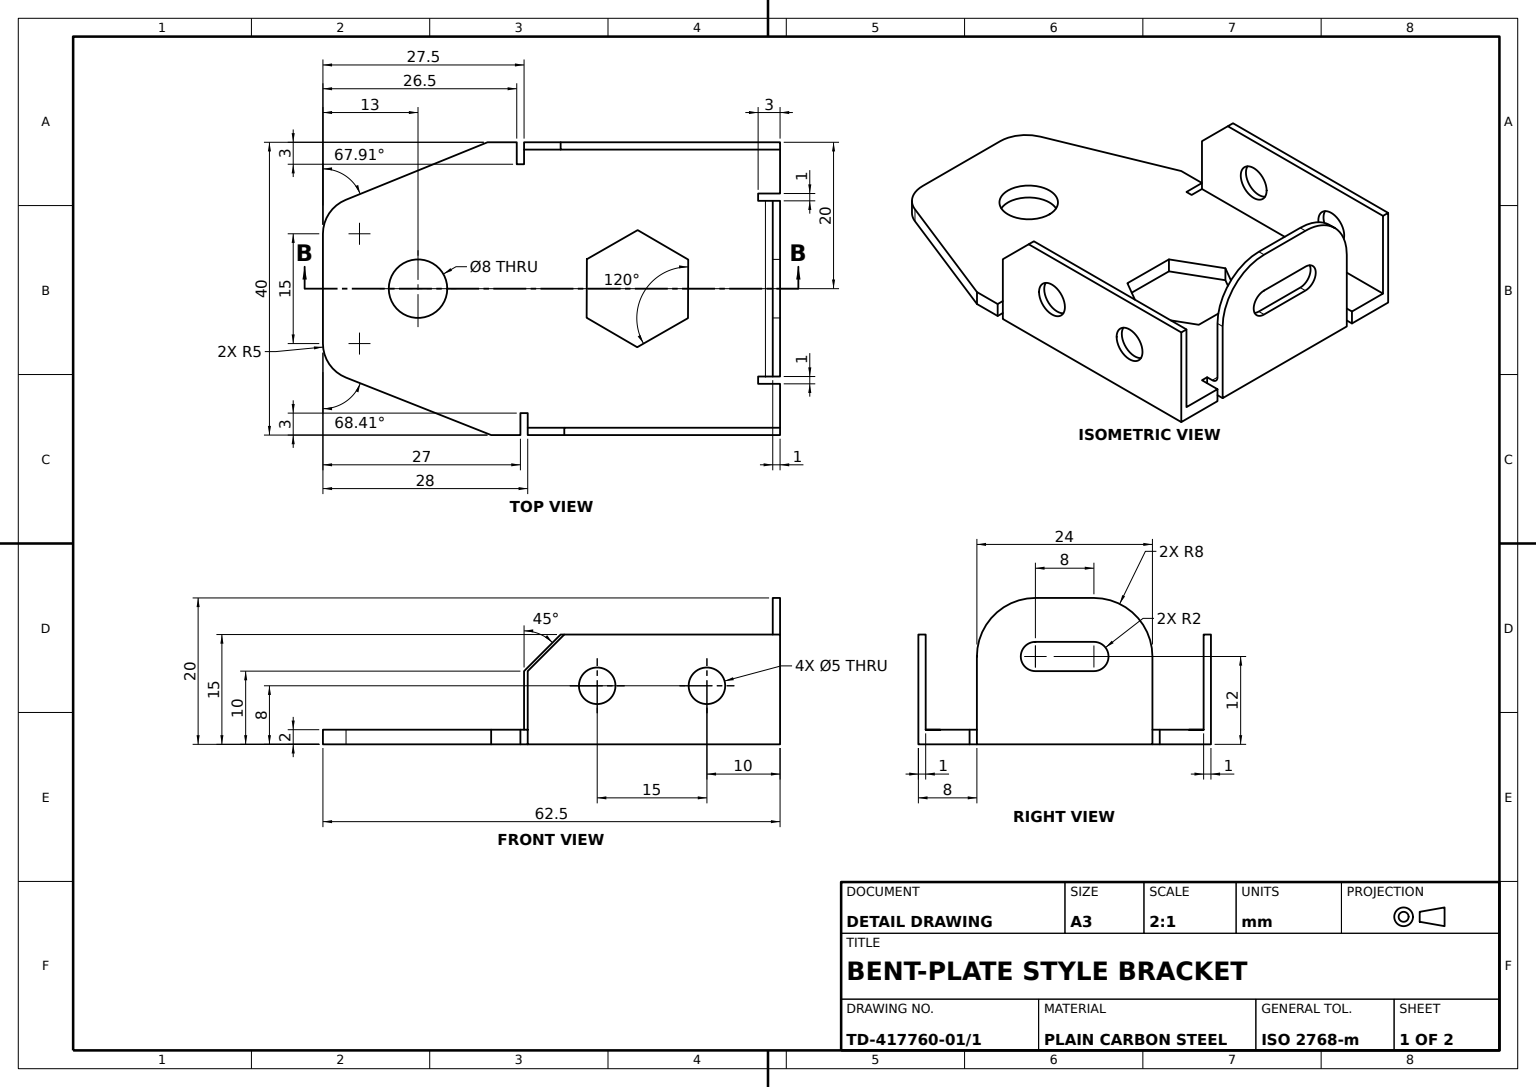
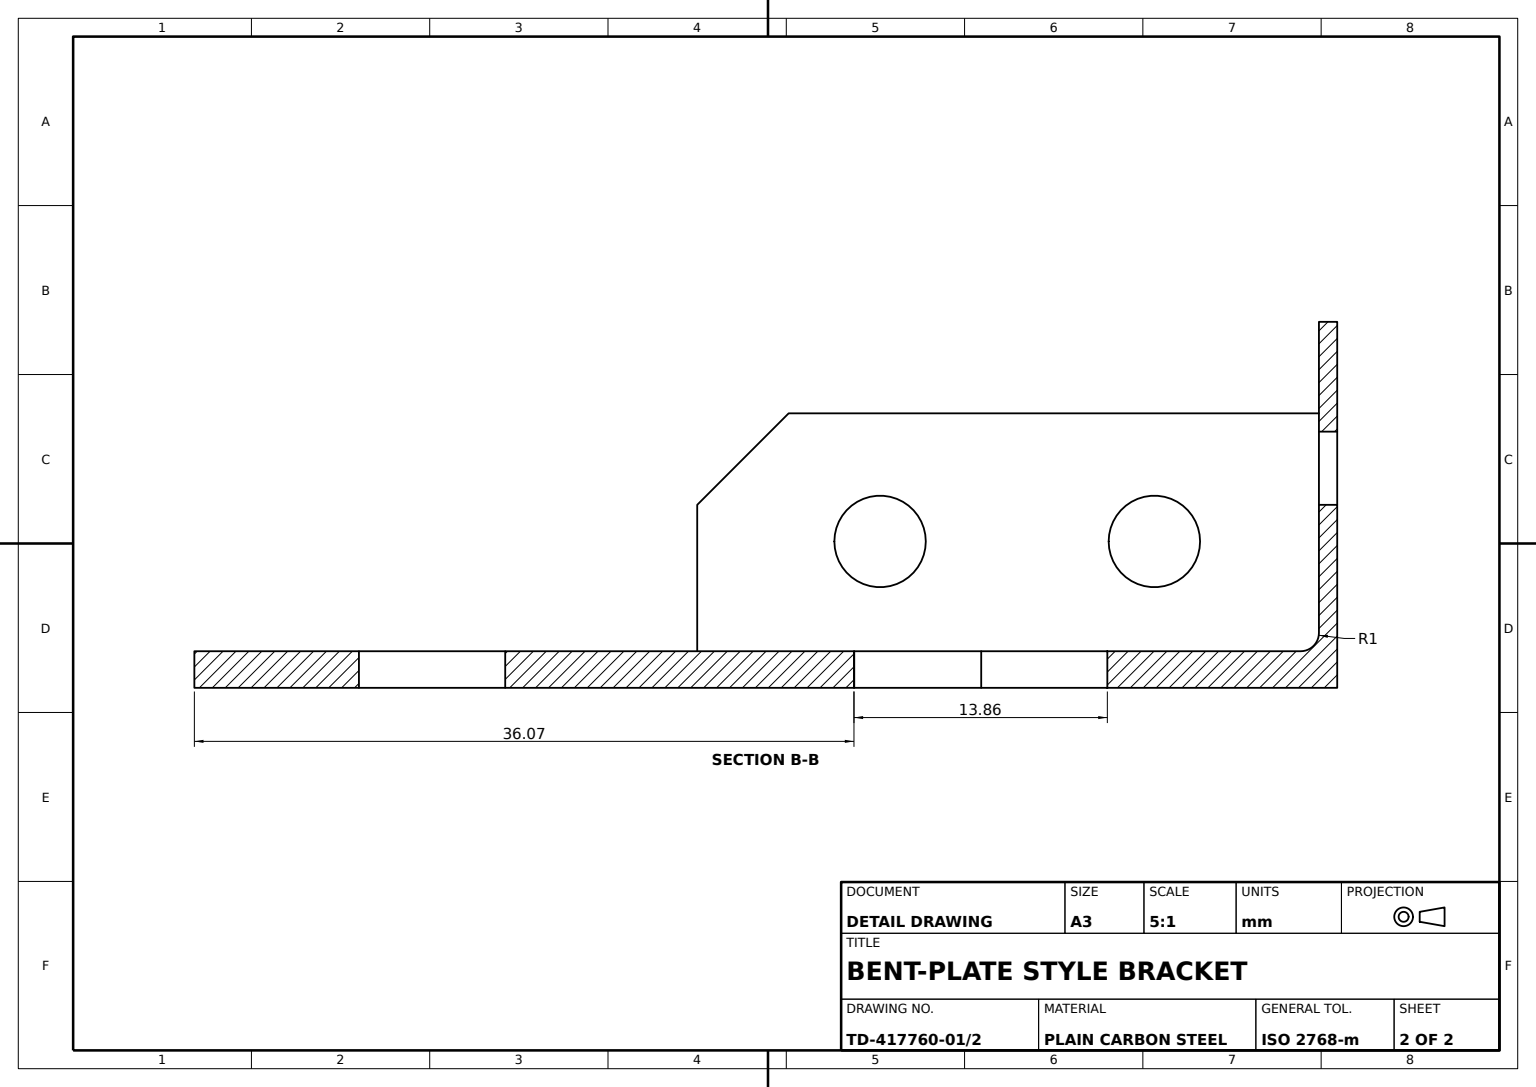
solid
v1 (4,20,1)
v2 (4,20,0)
e1 v1 v2 LINE
v3 (12,12,1)
e2 v3 v1 CIRCLE(AX(P(4,12,1),D(0,0,1),D(1,0,0)),8)
v4 (12,12,0)
e3 v4 v3 LINE
e4 v2 v4 CIRCLE(AX(P(4,12,0),D(0,0,-1),D(-1,0,0)),8)
face CYL(AX(P(4,12,1),D(0,0,-1),D(-1,0,0)),8) [-e1 -e2 -e3 -e4]
v5 (-3.99888,14,0)
v6 (3.99888,14,0)
e5 v5 v6 LINE
v7 (3.99888,14,1)
e6 v6 v7 LINE
v8 (-3.99888,14,1)
e7 v7 v8 LINE
e8 v5 v8 LINE
face PLANE(AX(P(-3.99888,14,-1),D(0,1,0),D(0,0,1))) rev [e5 e6 e7 -e8]
v9 (-19,2,35)
v10 (-17,2,35)
e9 v9 v10 LINE
v11 (-19,10,35)
e10 v9 v11 LINE
v12 (-20,10,35)
e11 v11 v12 LINE
v13 (-20,0,35)
e12 v12 v13 LINE
v14 (-17,0,35)
e13 v13 v14 LINE
e14 v10 v14 LINE
face PLANE(AX(P(0,2,35),D(0,0,-1),D(-1,0,0))) rev [-e9 e10 e11 e12 e13 -e14]
v15 (0,2,53.5)
v16 (0,2,45.5)
e15 v15 v16 CIRCLE(AX(P(0,2,49.5),D(0,1,0),D(0,0,1)),4)
v17 (0,0,45.5)
e16 v16 v17 LINE
v18 (0,0,53.5)
e17 v18 v17 CIRCLE(AX(P(0,0,49.5),D(0,1,0),D(0,0,1)),4)
e18 v15 v18 LINE
face CYL(AX(P(0,2,49.5),D(0,-1,0),D(0,0,-1)),4) rev [e15 e16 -e17 -e18]
v19 (3.973244,2,26.443651)
v20 (8,2,19.530895)
e19 v19 v20 LINE
v21 (8,0,19.530895)
e20 v20 v21 LINE
v22 (3.973244,0,26.443651)
e21 v22 v21 LINE
e22 v19 v22 LINE
face PLANE(AX(P(14.467771,2,8.427635),D(-0.864088023,0,-0.503340728),D(-0.503340728,0,0.864088023))) [e19 e20 -e21 -e22]
v23 (-20,8,27.5)
v24 (-20,8,22.5)
e23 v23 v24 CIRCLE(AX(P(-20,8,25),D(-1,0,0),D(0,0,1)),2.5)
e24 v24 v23 CIRCLE(AX(P(-20,8,25),D(-1,0,0),D(0,0,1)),2.5)
v25 (-20,8,12.5)
v26 (-20,8,7.5)
e25 v25 v26 CIRCLE(AX(P(-20,8,10),D(-1,0,0),D(0,0,1)),2.5)
e26 v26 v25 CIRCLE(AX(P(-20,8,10),D(-1,0,0),D(0,0,1)),2.5)
v27 (-20,15,0)
v28 (-20,0,0)
e27 v27 v28 LINE
e28 v28 v13 LINE
v29 (-20,15,30)
e29 v12 v29 LINE
e30 v29 v27 LINE
face PLANE(AX(P(-20,2,0),D(1,0,0),D(0,0,-1))) rev [-e23 -e24] [-e25 -e26] [e27 e28 -e12 e29 e30]
v30 (-8,2,19.469105)
v31 (-8,0,19.469105)
e31 v30 v31 LINE
v32 (-4.026756,2,26.412756)
e32 v30 v32 LINE
v33 (-4.026756,0,26.412756)
e33 v32 v33 LINE
e34 v31 v33 LINE
face PLANE(AX(P(-14.419221,2,8.250859),D(0.867949869,0,-0.496651815),D(-0.496651815,0,-0.867949869))) [-e31 e32 e33 -e34]
e35 v16 v15 CIRCLE(AX(P(0,2,49.5),D(0,1,0),D(0,0,1)),4)
e36 v17 v18 CIRCLE(AX(P(0,0,49.5),D(0,1,0),D(0,0,1)),4)
face CYL(AX(P(0,2,49.5),D(0,-1,0),D(0,0,-1)),4) rev [e35 e18 -e36 -e16]
v34 (20,15,0)
v35 (20,0,0)
e37 v34 v35 LINE
v36 (13,0,0)
e38 v36 v35 LINE
v37 (13,2,0)
e39 v37 v36 LINE
v38 (19,2,0)
e40 v37 v38 LINE
v39 (19,15,0)
e41 v38 v39 LINE
e42 v39 v34 LINE
face PLANE(AX(P(0,2,0),D(0,0,-1),D(-1,0,0))) [e37 -e38 -e39 e40 e41 e42]
v40 (4.026756,0,12.587244)
e43 v21 v40 LINE
v41 (4.026756,2,12.587244)
e44 v20 v41 LINE
e45 v41 v40 LINE
face PLANE(AX(P(-2.392465,2,1.368999),D(-0.867949869,0,0.496651815),D(0.496651815,0,0.867949869))) [-e43 -e20 e44 e45]
v42 (20,8,22.5)
v43 (20,8,27.5)
e46 v42 v43 CIRCLE(AX(P(20,8,25),D(1,0,0),D(0,0,-1)),2.5)
v44 (19,8,27.5)
e47 v43 v44 LINE
v45 (19,8,22.5)
e48 v45 v44 CIRCLE(AX(P(19,8,25),D(1,0,0),D(0,0,-1)),2.5)
e49 v42 v45 LINE
face CYL(AX(P(30,8,25),D(-1,0,0),D(0,0,1)),2.5) rev [e46 e47 -e48 -e49]
v46 (12,2,2)
v47 (12,2,3)
e50 v46 v47 LINE
v48 (-12,2,2)
e51 v46 v48 LINE
v49 (-12,2,3)
e52 v48 v49 LINE
v50 (-13,2,3)
e53 v49 v50 LINE
v51 (-13,2,0)
e54 v50 v51 LINE
v52 (-19,2,0)
e55 v52 v51 LINE
e56 v52 v9 LINE
v53 (-17,2,36)
e57 v10 v53 LINE
v54 (-20,2,36)
e58 v53 v54 LINE
v55 (-20,2,40)
e59 v54 v55 LINE
v56 (-12.132851,2,59.380608)
e60 v56 v55 LINE
v57 (-7.5,2,62.5)
e61 v56 v57 CIRCLE(AX(P(-7.5,2,57.5),D(0,1,0),D(0,0,1)),5)
v58 (7.5,2,62.5)
e62 v57 v58 LINE
v59 (12.14923,2,59.339743)
e63 v58 v59 CIRCLE(AX(P(7.5,2,57.5),D(0,1,0),D(0,0,1)),5)
v60 (20,2,39.5)
e64 v59 v60 LINE
v61 (20,2,35.5)
e65 v61 v60 LINE
v62 (17,2,35.5)
e66 v62 v61 LINE
v63 (17,2,34.5)
e67 v63 v62 LINE
v64 (19,2,34.5)
e68 v64 v63 LINE
e69 v64 v38 LINE
v65 (13,2,3)
e70 v65 v37 LINE
e71 v47 v65 LINE
v66 (-3.973244,2,12.556349)
e72 v66 v30 LINE
e73 v41 v66 LINE
e74 v32 v19 LINE
face PLANE(AX(P(0,2,0),D(0,1,0),D(0,0,1))) [-e50 e51 e52 e53 e54 -e55 e56 e9 e57 e58 e59 -e60 e61 e62 e63 e64 -e65 -e66 -e67 -e68 e69 -e40 -e70 -e71] [-e72 -e73 -e44 -e19 -e74 -e32] [-e35 -e15]
v67 (20,15,29.5)
v68 (20,10,34.5)
e75 v67 v68 LINE
v69 (19,15,29.5)
e76 v69 v67 LINE
v70 (19,10,34.5)
e77 v69 v70 LINE
e78 v70 v68 LINE
face PLANE(AX(P(19,22.25,22.25),D(0,0.707106781,0.707106781),D(0,-0.707106781,0.707106781))) [-e75 -e76 e77 e78]
v71 (-19,8,22.5)
e79 v71 v24 LINE
v72 (-19,8,27.5)
e80 v72 v71 CIRCLE(AX(P(-19,8,25),D(-1,0,0),D(0,0,1)),2.5)
e81 v72 v23 LINE
face CYL(AX(P(30,8,25),D(-1,0,0),D(0,0,1)),2.5) rev [e23 -e79 -e80 e81]
v73 (-4,20,0)
e82 v73 v2 LINE
v74 (-4,20,1)
e83 v73 v74 LINE
e84 v74 v1 LINE
face PLANE(AX(P(12,20,1),D(0,1,0),D(0,0,1))) [-e82 e83 e84 e1]
v75 (-20,0,40)
e85 v55 v75 LINE
v76 (-20,0,36)
e86 v54 v76 LINE
e87 v76 v75 LINE
face PLANE(AX(P(-20,2,0),D(1,0,0),D(0,0,-1))) rev [-e85 -e59 e86 e87]
v77 (20,8,7.5)
v78 (19,8,7.5)
e88 v77 v78 LINE
v79 (20,8,12.5)
e89 v77 v79 CIRCLE(AX(P(20,8,10),D(1,0,0),D(0,0,-1)),2.5)
v80 (19,8,12.5)
e90 v79 v80 LINE
e91 v78 v80 CIRCLE(AX(P(19,8,10),D(1,0,0),D(0,0,-1)),2.5)
face CYL(AX(P(30,8,10),D(-1,0,0),D(0,0,1)),2.5) rev [-e88 e89 e90 -e91]
v81 (12,3,1)
e92 v81 v46 CIRCLE(AX(P(12,3,2),D(-1,0,0),D(0,0,-1)),1)
v82 (-12,3,1)
e93 v82 v81 LINE
e94 v48 v82 CIRCLE(AX(P(-12,3,2),D(1,0,0),D(0,0,-1)),1)
face CYL(AX(P(0,3,2),D(-1,0,0),D(0,0,1)),1) rev [-e51 -e92 -e93 -e94]
e95 v43 v42 CIRCLE(AX(P(20,8,25),D(1,0,0),D(0,0,-1)),2.5)
e96 v79 v77 CIRCLE(AX(P(20,8,10),D(1,0,0),D(0,0,-1)),2.5)
e97 v34 v67 LINE
v83 (20,0,34.5)
e98 v68 v83 LINE
e99 v35 v83 LINE
face PLANE(AX(P(20,2,0),D(1,0,0),D(0,0,-1))) [-e95 -e46] [-e96 -e89] [-e37 e97 e75 e98 -e99]
e100 v44 v45 CIRCLE(AX(P(19,8,25),D(1,0,0),D(0,0,-1)),2.5)
e101 v64 v70 LINE
e102 v39 v69 LINE
e103 v80 v78 CIRCLE(AX(P(19,8,10),D(1,0,0),D(0,0,-1)),2.5)
face PLANE(AX(P(19,0,0),D(1,0,0),D(0,0,-1))) rev [e100 e48] [e101 -e77 -e102 -e41 -e69] [e91 e103]
v84 (-19,8,7.5)
e104 v84 v26 LINE
v85 (-19,8,12.5)
e105 v85 v84 CIRCLE(AX(P(-19,8,10),D(-1,0,0),D(0,0,1)),2.5)
e106 v85 v25 LINE
face CYL(AX(P(30,8,10),D(-1,0,0),D(0,0,1)),2.5) rev [e25 -e104 -e105 e106]
v86 (13,0,3)
e107 v65 v86 LINE
v87 (12,0,3)
e108 v87 v86 LINE
e109 v47 v87 LINE
face PLANE(AX(P(0,2,3),D(0,0,-1),D(-1,0,0))) [e107 -e108 -e109 e71]
v88 (-13,0,3)
v89 (-13,0,0)
e110 v88 v89 LINE
e111 v51 v89 LINE
e112 v50 v88 LINE
face PLANE(AX(P(-13,2,0),D(-1,0,0),D(0,0,1))) rev [e110 -e111 -e54 e112]
v90 (-17,0,36)
e113 v53 v90 LINE
e114 v90 v76 LINE
face PLANE(AX(P(0,2,36),D(0,0,1),D(1,0,0))) rev [e113 e114 -e86 -e58]
v91 (17,0,35.5)
e115 v62 v91 LINE
v92 (17,0,34.5)
e116 v92 v91 LINE
e117 v63 v92 LINE
face PLANE(AX(P(17,2,0),D(1,0,0),D(0,0,-1))) [e115 -e116 -e117 e67]
v93 (20,0,35.5)
e118 v61 v93 LINE
v94 (20,0,39.5)
e119 v60 v94 LINE
e120 v93 v94 LINE
face PLANE(AX(P(20,2,0),D(1,0,0),D(0,0,-1))) [-e118 e65 e119 -e120]
e121 v84 v85 CIRCLE(AX(P(-19,8,10),D(-1,0,0),D(0,0,1)),2.5)
e122 v71 v72 CIRCLE(AX(P(-19,8,25),D(-1,0,0),D(0,0,1)),2.5)
v95 (-19,15,30)
v96 (-19,15,0)
e123 v95 v96 LINE
e124 v11 v95 LINE
e125 v96 v52 LINE
face PLANE(AX(P(-19,0,0),D(-1,0,0),D(0,0,1))) rev [e121 e105] [e80 e122] [-e123 -e124 -e10 -e56 -e125]
v97 (7.5,0,62.5)
e126 v58 v97 LINE
v98 (-7.5,0,62.5)
e127 v57 v98 LINE
e128 v98 v97 LINE
face PLANE(AX(P(0,2,62.5),D(0,0,-1),D(-1,0,0))) rev [-e126 -e62 e127 e128]
v99 (-12,12,1)
e129 v82 v99 LINE
v100 (-12,12,0)
e130 v99 v100 LINE
v101 (-12,0,0)
e131 v101 v100 LINE
v102 (-12,0,3)
e132 v101 v102 LINE
e133 v49 v102 LINE
face PLANE(AX(P(-12,2,0),D(1,0,0),D(0,0,-1))) rev [-e52 e94 e129 e130 -e131 e132 -e133]
e134 v95 v29 LINE
face PLANE(AX(P(-19,10,35),D(0,0.707106781,0.707106781),D(0,-0.707106781,0.707106781))) [e124 e134 -e29 -e11]
e135 v86 v36 LINE
face PLANE(AX(P(13,2,0),D(-1,0,0),D(0,0,1))) [e70 e39 -e135 -e107]
face CYL(AX(P(30,8,10),D(-1,0,0),D(0,0,1)),2.5) rev [-e106 -e121 e104 e26]
v103 (-3.973244,0,12.556349)
e136 v66 v103 LINE
e137 v40 v103 LINE
face PLANE(AX(P(-0.04855,2,12.571506),D(-0.003861845,0,0.999992543),D(0.999992543,0,0.003861845))) [e73 e136 -e137 -e45]
e138 v102 v88 LINE
face PLANE(AX(P(0,2,3),D(0,0,1),D(1,0,0))) rev [e133 e138 -e112 -e53]
e139 v74 v99 CIRCLE(AX(P(-4,12,1),D(0,0,1),D(1,0,0)),8)
e140 v100 v73 CIRCLE(AX(P(-4,12,0),D(0,0,-1),D(-1,0,0)),8)
face CYL(AX(P(-4,12,0),D(0,0,1),D(1,0,0)),8) [-e139 -e83 -e140 -e130]
e141 v14 v90 LINE
face PLANE(AX(P(-17,2,0),D(1,0,0),D(0,0,-1))) rev [e141 -e113 -e57 e14]
v104 (-3.99888,10,0)
v105 (-3.99888,10,1)
e142 v104 v105 LINE
v106 (3.99888,10,1)
e143 v105 v106 LINE
v107 (3.99888,10,0)
e144 v107 v106 LINE
e145 v107 v104 LINE
face PLANE(AX(P(-3.99888,10,-1),D(0,-1,0),D(0,0,-1))) rev [e142 e143 -e144 e145]
v108 (5.99888,12,1)
e146 v108 v7 CIRCLE(AX(P(3.99888,12,1),D(0,0,1),D(1,0,0)),2)
e147 v106 v108 CIRCLE(AX(P(3.99888,12,1),D(0,0,1),D(1,0,0)),2)
e148 v8 v105 CIRCLE(AX(P(-3.99888,12,1),D(0,0,1),D(1,0,0)),2)
e149 v3 v81 LINE
face PLANE(AX(P(0,0,1),D(0,0,1),D(1,0,0))) [-e7 -e146 -e147 -e143 -e148] [e139 -e129 e93 -e149 e2 -e84]
face CYL(AX(P(30,8,25),D(-1,0,0),D(0,0,1)),2.5) rev [e79 e24 -e81 -e122]
e150 v91 v93 LINE
face PLANE(AX(P(0,2,35.5),D(0,0,-1),D(-1,0,0))) [e66 e118 -e150 -e115]
e151 v96 v27 LINE
face PLANE(AX(P(-19,15,30),D(0,1,0),D(0,0,1))) [-e30 -e134 e123 e151]
face CYL(AX(P(30,8,10),D(-1,0,0),D(0,0,1)),2.5) rev [-e90 e96 e88 -e103]
v109 (5.99888,12,0)
e152 v109 v107 CIRCLE(AX(P(3.99888,12,0),D(0,0,-1),D(-1,0,0)),2)
e153 v109 v108 LINE
face CYL(AX(P(3.99888,12,-1),D(0,0,1),D(1,0,0)),2) rev [e152 e144 e147 -e153]
e154 v103 v31 LINE
face PLANE(AX(P(2.494526,2,1.453089),D(0.864088023,0,0.503340728),D(0.503340728,0,-0.864088023))) [e31 -e154 -e136 e72]
v110 (-12.132851,0,59.380608)
e155 v110 v98 CIRCLE(AX(P(-7.5,0,57.5),D(0,1,0),D(0,0,1)),5)
e156 v56 v110 LINE
face CYL(AX(P(-7.5,2,57.5),D(0,-1,0),D(0,0,-1)),5) [e155 -e127 -e61 e156]
face PLANE(AX(P(19,15,0),D(0,1,0),D(0,0,1))) [e102 e76 -e97 -e42]
v111 (12.14923,0,59.339743)
e157 v59 v111 LINE
e158 v97 v111 CIRCLE(AX(P(7.5,0,57.5),D(0,1,0),D(0,0,1)),5)
face CYL(AX(P(7.5,2,57.5),D(0,-1,0),D(0,0,-1)),5) [-e157 -e63 e126 e158]
face CYL(AX(P(30,8,25),D(-1,0,0),D(0,0,1)),2.5) rev [e95 e49 -e100 -e47]
e159 v111 v94 LINE
face PLANE(AX(P(30.806633,2,12.190469),D(-0.929846099,0,-0.36794868),D(-0.36794868,0,0.929846099))) rev [e157 e159 -e119 -e64]
e160 v110 v75 LINE
face PLANE(AX(P(-31.110776,2,12.628762),D(-0.926570295,0,0.37612164),D(0.37612164,0,0.926570295))) [e60 e85 -e160 -e156]
v112 (12,0,0)
e161 v112 v87 LINE
e162 v4 v112 LINE
face PLANE(AX(P(12,2,0),D(1,0,0),D(0,0,-1))) [e92 e50 e109 -e161 -e162 e3 e149]
e163 v28 v89 LINE
face PLANE(AX(P(0,2,0),D(0,0,-1),D(-1,0,0))) [e111 -e163 -e27 -e151 e125 e55]
e164 v6 v109 CIRCLE(AX(P(3.99888,12,0),D(0,0,-1),D(-1,0,0)),2)
face CYL(AX(P(3.99888,12,-1),D(0,0,1),D(1,0,0)),2) rev [e164 e153 e146 -e6]
e165 v33 v22 LINE
face PLANE(AX(P(-0.102061,2,26.427912),D(0.003861845,0,-0.999992543),D(-0.999992543,0,-0.003861845))) [-e33 e74 e22 -e165]
e166 v104 v5 CIRCLE(AX(P(-3.99888,12,0),D(0,0,-1),D(-1,0,0)),2)
face CYL(AX(P(-3.99888,12,-1),D(0,0,1),D(1,0,0)),2) rev [e166 e8 e148 -e142]
e167 v83 v92 LINE
face PLANE(AX(P(0,2,34.5),D(0,0,1),D(1,0,0))) [-e78 -e101 e68 e117 -e167 -e98]
e168 v112 v101 LINE
face PLANE(AX(P(0,0,0),D(0,1,0),D(0,0,1))) rev [e17 e36] [e21 e43 e137 e154 e34 e165] [e120 -e159 -e158 -e128 -e155 e160 -e87 -e114 -e141 -e13 -e28 e163 -e110 -e138 -e132 -e168 e161 e108 e135 e38 e99 e167 e116 e150]
face PLANE(AX(P(0,0,0),D(0,0,-1),D(-1,0,0))) [e140 e82 e4 e162 e168 e131] [-e145 -e152 -e164 -e5 -e166]
